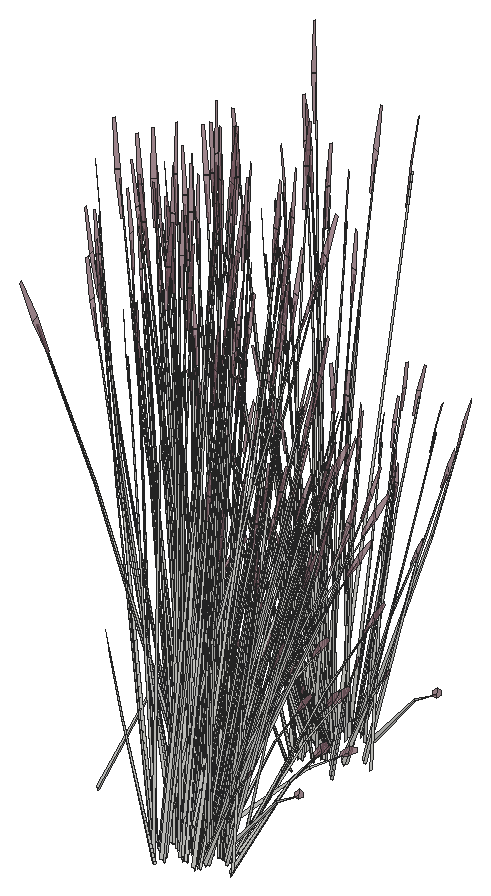
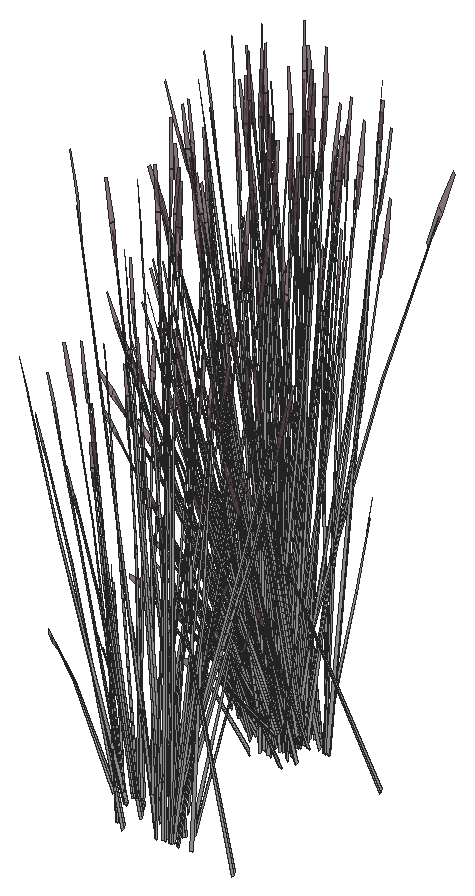
# SketchUp Ruby script. Lengths in inches.
U = 1.inch
M = Sketchup.active_model
def pt(a) = Geom::Point3d.new(a.map { |v| v * U })
def face(e, loops, mat)
  f = e.add_face(loops[0].map { |a| pt(a) })
  loops[1..].each { |l| e.add_face(l.map { |a| pt(a) }).erase! }
  f.material = f.back_material = mat if mat
  f
end
# faces: each face lists its corners as indices into pts; further lists are holes
def faces(e, pts, list, mat = nil) = list.each { |f| face(e, (f[0].is_a?(Array) ? f : [f]).map { |l| l.map { |i| pts[i] } }, mat) }
# xy, xz, yz: faces in a plane at the given z, y or x. An outline is a flat list of corners, or four numbers for a rectangle; further outlines are holes
def ring(l) = l.size == 4 ? [[l[0], l[1]], [l[2], l[1]], [l[2], l[3]], [l[0], l[3]]] : l.each_slice(2).to_a
def flat(e, list, mat, &to3) = list.each { |f| face(e, (f[0].is_a?(Array) ? f : [f]).map { |l| ring(l).map { |u, v| to3.(u, v) } }, mat) }
def xy(e, z, list, mat = nil) = flat(e, list, mat) { |x, y| [x, y, z] }
def xz(e, y, list, mat = nil) = flat(e, list, mat) { |x, z| [x, y, z] }
def yz(e, x, list, mat = nil) = flat(e, list, mat) { |y, z| [x, y, z] }
def lines(e, pts, list) = list.each { |a, b| e.add_line(pt(pts[a]), pt(pts[b])) }
# prism: a flat outline (further loops are holes) pulled along v
def prism(e, loops, v, mat = nil)
  f = face(e, loops, mat); d = Geom::Vector3d.new(v.map { |x| x * U })
  f.pushpull(f.normal.samedirection?(d) ? d.length : -d.length)
end
def box(e, o, s, mat = nil) = prism(e, [[o, [o[0] + s[0], o[1], o[2]], [o[0] + s[0], o[1] + s[1], o[2]], [o[0], o[1] + s[1], o[2]]]], [0, 0, s[2]], mat)
def at(x, y, z, deg = 0) = Geom::Transformation.translation(pt([x, y, z])) * Geom::Transformation.rotation(ORIGIN, Z_AXIS, deg.degrees)
def axes(o, x, y, z) = Geom::Transformation.new([*x, 0, *y, 0, *z, 0, *pt(o).to_a, 1])
def part(name) = M.definitions.add(name)
# library, detail: a bought-in or finely detailed component or shape, given as its bounding box
def library(name, o, s) = part(name).tap { |d| box(d.entities, o, s) }
def detail(e, o, s) = box(e.add_group.entities, o, s)
def put(e, d, t, mat = nil) = e.add_instance(d, t).tap { |i| i.material = mat if mat }
def group(e, t, mat = nil) = e.add_group.tap { |g| g.transformation = t; g.material = mat if mat }.entities
root = M.entities
M.materials.add("LightPink_Translucent").color = [144, 107, 117]
M.materials["LightPink_Translucent"].alpha = 0.75
c1 = part("blade")
p = [[2.15,0.21,22],[0,0.17,0],[0.09,0.45,0],[2.18,0.31,22],[2.29,0.31,22],[0.38,0.45,0],
  [2.48,0.24,33],[2.49,0.24,33],[2.48,0.22,33]]
faces(c1.entities,p,[[0,1,2,3],[4,5,2,3],[6,3,4,7],[8,0,3,6]])
c2 = part("seeds")
p = [[0.3,-0.1,1.38],[-0.01,-0.03,1.59],[-0.01,-0.03,0.03],[0.14,-0.07,-0.07],[0.29,-0.03,3],[0.15,0.01,3.11]]
faces(c2.entities,p,[[0,1,2,3],[1,0,4,5]],"LightPink_Translucent")
c3 = part("blade with seeds")
put(c3.entities,c1,at(0,0,0))
put(c3.entities,c2,axes([2.4,0.25,30.99],[1.5799,-0.05474,1.17369],[-0.12525,1.92788,0.29478],[-0.07173,-0.02425,1.56792]))
put(root,c3,axes([506.375,142.96,1.57],[-0.47504,-0.61229,0],[0.79476,-0.34146,-0.51607],[0.18101,-0.07777,1.63711]))
put(root,c3,axes([510.65,144.14,3.875],[-0.19519,-0.55794,-0.51099],[0.73919,-0.0976,-0.3958],[0.21183,-0.14986,0.97773]))
put(root,c3,axes([507.42,142.22,1.32],[-0.52505,0.35054,-0.03893],[-0.48109,-0.38392,-0.17649],[-0.03387,-0.10878,0.58215]))
put(root,c3,axes([510.99,144.54,4.23],[-0.70283,-0.33692,-0.1216],[0.40491,-0.48793,-0.67495],[0.19857,-0.16961,1.02557]))
put(root,c3,axes([508.09,146.38,2.52],[0.65659,0.2464,1.51261],[-0.64324,0.53082,0.59816],[-0.28812,-0.31461,1.26806]))
put(root,c3,axes([504.66,144.68,1.21],[0,-0.61104,-0.49651],[0.85008,0,0],[0,-0.13917,1.57504]))
put(root,c3,axes([507.02,142.87,1.21],[0.7111,-0.30552,-0.49651],[0.42504,0.54784,0],[0.16196,-0.06958,1.57504]))
put(root,c3,axes([511.24,143.92,1.78],[-0.27143,-0.0181,1.43002],[-0.27808,-0.48551,-0.30754],[0.33346,-0.13735,0.61141]))
put(root,c3,axes([512.72,144.39,3.9],[-0.09924,-0.00464,1.77383],[-0.4121,-0.49725,-0.16761],[0.1655,-0.1635,0.31391]))
put(root,c3,axes([507.86,144.12,1.25],[0.51177,-0.45928,-0.62353],[0.63575,0.41646,-0.16365],[0.20507,-0.11457,1.37633]))
put(root,c3,axes([511.55,143.03,1.96],[-0.25308,0.31105,1.1486],[-0.21753,-0.4179,0.84392],[0.20902,-0.10472,0.25299]))
put(root,c3,axes([511.19,144.2,3.72],[0.66138,-0.08733,-0.35414],[0.17464,0.49921,0.4572],[0.18953,-0.13408,0.87481]))
put(root,c3,axes([506.97,144.93,1.4],[0.36864,-0.55059,-0.44739],[0.76598,0.26498,0.21531],[0,-0.12692,1.43643]))
put(root,c3,axes([507.31,144.65,1.86],[-0.08854,-0.69723,-0.29095],[0.92215,-0.04216,-0.50002],[0.16238,-0.09287,1.59708]))
put(root,c3,axes([505.02,144.69,1.22],[0.53038,-0.38124,-0.30978],[0.53038,0.38124,0.30978],[0,-0.1228,1.38974]))
put(root,c3,axes([510.65,144.49,4.24],[-0.66138,0.08733,0.35414],[-0.17464,-0.49921,-0.4572],[0.18953,-0.13408,0.87481]))
put(root,c3,axes([506.88,145.38,1.86],[-0.85568,-0.29155,-0.29095],[0.41201,-0.61537,-0.50002],[-0.02689,-0.15109,1.59708]))
put(root,c3,axes([507.1875,143.11,1.22],[0.70886,0.15119,-0.30978],[-0.17848,0.53243,0.30978],[0.1429,-0.0614,1.38974]))
put(root,c3,axes([511.25,144.42,3.92],[0.52161,0.25698,0.0643],[-0.30368,0.36595,0.50621],[0.16723,-0.11831,0.77189]))
put(root,c3,axes([511.11,144.31,3.93],[0.18844,0.56237,0.48003],[-0.73919,0.0976,0.3958],[0.21785,-0.13226,0.9933]))
put(root,c3,axes([513.1,144.99,3.91],[0.10543,-0.09307,1.74944],[-0.13495,-0.57092,-0.27667],[0.26455,-0.10825,0.14031]))
put(root,c3,axes([505.18,144.96,1.52],[-0.70674,0.51372,0.30756],[-0.70717,-0.50832,-0.36492],[-0.02468,-0.14589,1.64885]))
put(root,c3,axes([507.43,145.2,1.625],[0.8561,0.29616,0.24065],[-0.41201,0.61537,0.50002],[0,-0.14185,1.60543]))
put(root,c3,axes([507.1,146.03,1.63],[0.20138,-0.72405,-0.23429],[0.95485,0.12621,0.51271],[-0.16685,-0.09999,1.5644]))
put(root,c3,axes([507.15,144.79,1.91],[-0.82508,0.03772,0.44739],[-0.07462,-0.62614,-0.21531],[0.14771,-0.06346,1.43643]))
put(root,c3,axes([505.02,145.24,1.67],[0,0.61104,0.49651],[-0.85008,0,0],[0,-0.13917,1.57504]))
put(root,c3,axes([511.02,145.86,4.23],[-0.38229,-0.5533,-0.1216],[0.6785,-0.2719,-0.67495],[0.28593,-0.073,1.02557]))
put(root,c3,axes([510.99,145.38,3.875],[0.20584,-0.55581,-0.51099],[0.70573,0.19051,-0.3958],[0.28414,-0.05097,0.97773]))
put(root,c3,axes([509.875,143.12,1.57],[0.47504,-0.61229,0],[0.79476,0.34146,-0.51607],[0.18101,0.07777,1.63711]))
put(root,c3,axes([507.03,145.74,1.4],[-0.45644,-0.51287,-0.44739],[0.69137,-0.36116,0.21531],[-0.14771,-0.06346,1.43643]))
put(root,c3,axes([507.125,145.01,1.55],[0.33034,0.68327,0.45755],[-0.94388,0.2376,0.17955],[0.01154,-0.12555,1.58856]))
put(root,c3,axes([511.74,145.54,1.17],[-0.48937,0.07333,1.41583],[-0.07789,-0.58369,0.08104],[0.34275,-0.08835,0.80566]))
put(root,c3,axes([512.63,145.02,1.45],[-0.47106,-0.39072,-0.06488],[0.51591,-0.35801,-0.29416],[0.14618,-0.02521,0.97024]))
put(root,c3,axes([506.96,145.55,1.91],[-0.36864,0.55059,0.44739],[-0.76598,-0.26498,-0.21531],[0,-0.12692,1.43643]))
put(root,c3,axes([508.3125,145.07,1.4],[0,-0.70701,0],[0.95008,0,0],[0,0,1.79456]))
put(root,c3,axes([509.46,143.4375,1.67],[-0.7111,-0.30552,0.49651],[0.42504,-0.54784,0],[0.16196,0.06958,1.57504]))
put(root,c3,axes([510.85,145.58,4.17],[0.66765,-0.26986,-0.71045],[0.37208,0.55551,0.08574],[0.32259,-0.0631,1.00501]))
put(root,c3,axes([507.86,144.625,1.55],[-0.62999,0.55453,0.45755],[-0.74845,-0.4895,0.17955],[0.15188,-0.05534,1.58856]))
put(root,c3,axes([508.55,145.62,1.49],[-0.70674,-0.52593,-0.06131],[0.70717,-0.52625,0],[-0.02468,-0.01837,1.75571]))
put(root,c3,axes([506.77,143.71,1.67],[-0.21949,0.60727,0.17642],[-0.8032,-0.17185,0.35086],[0.13875,-0.00296,1.60407]))
put(root,c3,axes([510.76,145.6875,4.24],[-0.63144,-0.17046,0.35414],[0.18417,-0.49731,-0.4572],[0.25423,-0.0456,0.87481]))
put(root,c3,axes([506.4375,144.2,0.79],[-0.74787,0.24464,1.28929],[-0.23804,-0.70192,0.50096],[0.45924,0.01168,1.46642]))
put(root,c3,axes([508.45,144.39,1.81],[0.14658,-0.54532,0.1448],[0.71613,0.09466,-0.41347],[0.13033,0.05599,1.26744]))
put(root,c3,axes([507.21,145.68,1.55],[0.96033,0.12874,0.45755],[-0.19544,0.7271,0.17955],[-0.14034,-0.07021,1.58856]))
put(root,c3,axes([512.28,145.16,0.6875],[-0.03971,-0.09277,1.76342],[0.27541,-0.54264,-0.26939],[0.27782,-0.00781,0.30037]))
put(root,c3,axes([508.14,144.53,1.91],[-0.45644,-0.51287,0.44739],[0.69137,-0.36116,-0.21531],[0.14771,0.06346,1.43643]))
put(root,c3,axes([506.69,146.84,1.67],[0.81646,-0.16218,0.17642],[0.20161,0.60355,0.35086],[-0.07282,-0.08794,1.60407]))
put(root,c3,axes([508.37,144.5625,1.86],[0.76714,-0.40567,-0.29095],[0.51013,0.57321,-0.50002],[0.18927,0.05821,1.59708]))
put(root,c3,axes([511.42,145.63,3.72],[0.63144,0.17046,-0.35414],[-0.18417,0.49731,0.4572],[0.25423,-0.0456,0.87481]))
put(root,c3,axes([510.31,143.49,1.21],[0.7111,0.30552,-0.49651],[-0.42504,0.54784,0],[0.16196,0.06958,1.57504]))
put(root,c3,axes([508.96,145.23,1.4],[0.85008,0,0],[0,0.63259,0],[0,0,1.78407]))
put(root,c3,axes([509.2,143.74,1.67],[-0.81646,0.16218,0.17642],[-0.20161,-0.60355,0.35086],[0.07282,0.08794,1.60407]))
put(root,c3,axes([509.7,145.02,3.07],[-0.31515,0.01384,1.71376],[0.20907,-0.5998,0.13857],[0.44912,0.0371,0.73262]))
put(root,c3,axes([510.11,143.71,1.22],[0.17848,0.53243,-0.30978],[-0.70886,0.15119,0.30978],[0.1429,0.0614,1.38974]))
put(root,c3,axes([511.33,145.84,3.92],[0.27906,0.41663,0.0643],[-0.50888,0.20393,0.50621],[0.22432,-0.04024,0.77189]))
put(root,c3,axes([508.68,144.91,1.57],[-0.96033,-0.12874,0.49198],[0.19544,-0.7271,0.19306],[0.14034,0.07021,1.70813]))
put(root,c3,axes([511.28,145.7,3.93],[-0.21466,0.55714,0.48003],[-0.70573,-0.19051,0.3958],[0.27753,-0.03348,0.9933]))
put(root,c3,axes([507.92,146.7,1.4],[-0.24791,-0.5268,0],[0.70791,-0.18448,0],[0,0,1.54371]))
put(root,c3,axes([507.44,146.2,1.81],[-0.14658,0.54532,0.1448],[-0.71613,-0.09466,-0.41347],[-0.13033,-0.05599,1.26744]))
put(root,c3,axes([508.84,146.63,1.38],[0.79769,-0.20732,-0.19198],[0.2803,0.59721,0.00008],[0.08805,-0.02292,1.73897]))
put(root,c3,axes([509.12,146.875,1.67],[0.21949,-0.60727,0.17642],[0.8032,0.17185,0.35086],[-0.13875,0.00296,1.60407]))
put(root,c3,axes([508.9375,145.5,1.41],[0.53038,0.39469,0],[-0.53038,0.39469,0],[0,0,1.69266]))
put(root,c3,axes([510.375,145.33,1.67],[-0.59697,-0.44509,0.17642],[0.60159,-0.4317,0.35086],[-0.06593,0.0909,1.60407]))
put(root,c3,axes([509.27,144.66,1.25],[0.79037,0.10018,-0.62353],[-0.16679,0.61794,-0.16365],[0.23587,0.07488,1.37633]))
put(root,c3,axes([512.76,145.73,1.96],[-0.46945,0.10088,1.1486],[0.22097,-0.4169,0.84392],[0.24904,0.02853,0.25299]))
put(root,c3,axes([507.74,146.94,1.39],[-0.76598,-0.27433,0],[0.36864,-0.57001,0],[0,0,1.62707]))
put(root,c3,axes([508.38,146.21,1.66],[-0.74193,-0.49181,-0.25192],[0.6243,-0.55226,0.5513],[-0.19979,0.05753,1.68216]))
put(root,c3,axes([506.42,147.15,1.67],[0.7111,0.30552,0.49651],[-0.42504,0.54784,0],[-0.16196,-0.06958,1.57504]))
put(root,c3,axes([508.93,145.04,1.91],[0.36864,-0.55059,0.44739],[0.76598,0.26498,-0.21531],[0,0.12692,1.43643]))
put(root,c3,axes([512.54,147.5,3.9],[-0.0687,-0.05349,1.77383],[0.15029,-0.57341,-0.16761],[0.27062,-0.03664,0.31391]))
put(root,c3,axes([508.79,145.35,1.48],[0,0.70667,-0.05637],[-0.95008,0,0],[0,0.02221,1.79368]))
put(root,c3,axes([508.86,144.85,1.4],[0.45644,0.51287,-0.44739],[-0.69137,0.36116,0.21531],[0.14771,0.06346,1.43643]))
put(root,c3,axes([511.95,147.02,3.12],[-0.14542,-0.51365,-0.03492],[0.68734,-0.11809,-0.15832],[0.14353,0.03256,0.52218]))
put(root,c3,axes([510.16,147,4.23],[0.04068,-0.62141,-0.1216],[0.77029,0.01698,-0.67495],[0.29667,0.04317,1.02557]))
put(root,c3,axes([510.87,145.34,1.67],[0,-0.61104,0.49651],[0.85008,0,0],[0,0.13917,1.57504]))
put(root,c3,axes([508.74,145.8,1.91],[0.82508,-0.03772,0.44739],[0.07462,0.62614,-0.21531],[-0.14771,0.06346,1.43643]))
put(root,c3,axes([509.25,145.16,1.81],[0.70791,-0.1782,0.1448],[0.24791,0.50885,-0.41347],[0,0.11199,1.26744]))
put(root,c3,axes([510.05,146.76,4.24],[-0.43232,-0.38257,0.35414],[0.49364,-0.36215,-0.4572],[0.25081,0.0551,0.87481]))
put(root,c3,axes([508,146.11,1.4],[-0.82508,0.03772,-0.44739],[-0.07462,-0.62614,0.21531],[-0.14771,0.06346,1.43643]))
put(root,c3,axes([511.88,146.4,1.78],[-0.18299,-0.15028,1.43002],[0.23809,-0.49714,-0.30754],[0.37023,0.06735,0.61141]))
put(root,c3,axes([508.61,146.95,1.4],[0.76598,0.27433,0],[-0.36864,0.57001,0],[0,0,1.74954]))
put(root,c3,axes([510.83,146.63,3.91],[0.16299,-0.01033,1.74944],[0.44707,-0.47471,-0.27667],[0.28992,0.06266,0.14031]))
put(root,c3,axes([508.92,147.56,1.39],[-0.46912,-0.61443,-0.05142],[0.79476,-0.34146,0.51607],[-0.19584,0.0585,1.6363]))
put(root,c3,axes([508.75,146.07,1.81],[0.56134,0.36712,0.1448],[-0.46823,0.41419,-0.41347],[-0.13033,0.05599,1.26744]))
put(root,c3,axes([510.2,146.71,4.17],[0.75952,0.01471,-0.71045],[-0.05101,0.61953,0.08574],[0.32177,0.06538,1.00501]))
put(root,c3,axes([509.35,147.2,1.67],[0.7111,-0.30552,0.49651],[0.42504,0.54784,0],[-0.16196,0.06958,1.57504]))
put(root,c3,axes([508.34,146.72,1.48],[0.33034,0.70197,-0.06012],[-0.94388,0.24598,0],[0.01154,0.02451,1.72173]))
put(root,c3,axes([508.7,147.48,1.22],[-0.70886,-0.15119,-0.30978],[0.17848,-0.53243,0.30978],[-0.1429,0.0614,1.38974]))
put(root,c3,axes([511.44,145.45,1.57],[0.95008,0,0],[0,0.68292,-0.51607],[0,0.15554,1.63711]))
put(root,c3,axes([511.0625,145.8,1.39],[-0.94962,-0.00489,-0.04976],[0,-0.68292,0.49943],[-0.02984,0.15546,1.58352]))
put(root,c3,axes([509.01,145.21,1.86],[0.85568,0.29155,-0.29095],[-0.41201,0.61537,-0.50002],[0.02689,0.15109,1.59708]))
put(root,c3,axes([510.66,146.96,3.72],[0.43232,0.38257,-0.35414],[-0.49364,0.36215,0.4572],[0.25081,0.0551,0.87481]))
put(root,c3,axes([510.87,145.9,1.22],[-0.53038,0.38124,-0.30978],[-0.53038,-0.38124,0.30978],[0,0.1228,1.38974]))
put(root,c3,axes([508.58,145.94,1.86],[0.08854,0.69723,-0.29095],[-0.92215,0.04216,-0.50002],[-0.16238,0.09287,1.59708]))
put(root,c3,axes([510.4375,147.11,3.92],[-0.03826,0.46465,0.0643],[-0.57772,-0.01274,0.50621],[0.2213,0.04862,0.77189]))
put(root,c3,axes([508.92,145.66,1.4],[-0.36864,0.55059,-0.44739],[-0.76598,-0.26498,0.21531],[0,0.12692,1.43643]))
put(root,c3,axes([497.1875,147.83,1.78],[-0.18299,-0.15028,1.43002],[0.23809,-0.49714,-0.30754],[0.37023,0.06735,0.61141]))
put(root,c3,axes([510.49,146.96,3.93],[-0.56024,0.40262,0.48003],[-0.48318,-0.42758,0.3958],[0.26285,0.07427,0.9933]))
put(root,c3,axes([508.71,147.43,4.24],[-0.11735,-0.49217,0.35414],[0.67083,-0.12996,-0.4572],[0.18018,0.14104,0.87481]))
put(root,c3,axes([508.9375,147.24,1.52],[0.95122,0.19861,0.30756],[-0.23797,0.7099,-0.36492],[-0.15744,0.08885,1.64885]))
put(root,c3,axes([508.87,147.72,1.21],[-0.7111,0.30552,-0.49651],[-0.42504,-0.54784,0],[-0.16196,0.06958,1.57504]))
put(root,c3,axes([511.23,145.91,1.21],[0,0.61104,-0.49651],[-0.85008,0,0],[0,0.13917,1.57504]))
put(root,c3,axes([509.11,145.98,3.07],[-0.28223,-0.10528,1.71376],[0.58406,-0.44165,0.13857],[0.36402,0.19924,0.73262]))
put(root,c3,axes([509.16,144.59,3.67],[-0.65655,-0.31748,1.38283],[0.69326,-0.49431,0.59665],[0.21183,0.29789,1.33663]))
put(root,c3,axes([510.15,147.18,1.96],[-0.4278,-0.1757,1.1486],[0.5524,-0.17852,0.84392],[0.14899,0.15122,0.25299]))
put(root,c3,axes([508.65,147.68,4.23],[0.45276,-0.52302,-0.1216],[0.65568,0.30132,-0.67495],[0.22792,0.14777,1.02557]))
put(root,c3,axes([505.66,146.97,4.24],[0.5141,-0.32171,0.35414],[0.48666,0.36734,-0.4572],[-0.07405,0.18664,0.87481]))
put(root,c3,axes([509.51,147.625,1.57],[0.47504,0.61229,0],[-0.79476,0.34146,-0.51607],[-0.18101,0.07777,1.63711]))
put(root,c3,axes([508.06,148.11,3.9],[0.00225,-0.07398,1.77383],[0.65113,-0.32638,-0.16761],[0.22617,0.1165,0.31391]))
put(root,c3,axes([510.27,147.83,0.6875],[0.05536,-0.08822,1.76342],[0.69692,-0.25981,-0.26939],[0.21129,0.13447,0.30037]))
put(root,c3,axes([509.11,145.2,2.03],[-0.02076,-0.57531,1.41272],[0.93937,0.14913,0.59816],[-0.22217,0.31481,1.3335]))
put(root,c3,axes([509.35,145.83,1.29],[0.2786,0.55945,-0.69212],[-0.80253,0.20149,-0.18165],[0.03079,0.18945,1.52773]))
put(root,c3,axes([509.18,147.42,3.875],[0.74975,-0.14525,-0.51099],[0.13115,0.55007,-0.3958],[0.20138,0.15763,0.97773]))
put(root,c3,axes([507.1,147.5,4.24],[0.22906,-0.4699,0.35414],[0.66828,0.13705,-0.4572],[0.06128,0.18919,0.87481]))
put(root,c3,axes([510.22,147.98,1.86],[-0.48723,-0.01916,1.0506],[0.32177,-0.40701,0.58006],[0.19248,0.1446,0.8241]))
put(root,c3,axes([508.82,147.87,3.92],[-0.34533,0.38816,0.0643],[-0.49176,-0.22599,0.50621],[0.15898,0.12445,0.77189]))
put(root,c3,axes([508,149.18,4.84],[0.52505,-0.35054,-0.06488],[0.48109,0.38392,-0.29416],[0.03387,0.10878,0.97024]))
put(root,c3,axes([508.96,147.76,3.93],[-0.75571,0.14023,0.48003],[-0.13115,-0.55007,0.3958],[0.17773,0.16212,0.9933]))
put(root,c3,axes([508.63,146.99,1.78],[0.01341,-0.20255,1.43002],[0.64074,-0.22625,-0.30754],[0.1978,0.24243,0.61141]))
put(root,c3,axes([506.9,147.93,3.92],[-0.55987,0.20767,0.0643],[-0.27403,-0.37869,0.50621],[0.05407,0.16693,0.77189]))
put(root,c3,axes([505.34,147.0625,4.59],[0.83505,0.03027,-0.13498],[-0.02282,0.57322,-0.74919],[-0.05801,0.22077,1.13838]))
put(root,c3,axes([506.88,147.7,4.23],[0.74352,-0.28449,-0.1216],[0.36538,0.50492,-0.67495],[0.0981,0.21277,1.02557]))
put(root,c3,axes([507.1,147.89,4.26],[-0.74868,-0.15974,0.53283],[0.25601,-0.52518,0.43934],[0.04499,0.20653,1.10256]))
put(root,c3,axes([505.72,148.68,1.96],[-0.01966,-0.36332,1.1486],[0.49135,0.25914,0.84392],[-0.09663,0.17317,0.25299]))
put(root,c3,axes([507.02,147.8125,0.6875],[0.12297,-0.03325,1.76342],[0.73967,0.18301,-0.26939],[0.02163,0.20626,0.30037]))
put(root,c3,axes([505.91,147.28,4.2],[0.54391,0.41056,-0.5672],[-0.57458,0.35956,-0.43934],[-0.08276,0.2086,1.08528]))
put(root,c3,axes([505.32,147.9,2.02],[0.69024,-0.1082,0.06507],[0.15868,0.43593,-0.86304],[-0.04376,0.22067,0.7736]))
put(root,c3,axes([507.52,147.68,3.875],[0.7469,0.15318,-0.51099],[-0.25601,0.52518,-0.3958],[0.06849,0.21144,0.97773]))
put(root,c3,axes([507.94,146.59,3.07],[-0.17368,-0.19618,1.71376],[0.80256,-0.16516,0.13857],[0.18139,0.30799,0.73262]))
put(root,c3,axes([507.18,148,3.72],[-0.22906,0.4699,-0.35414],[-0.66828,-0.13705,0.4572],[0.06128,0.18919,0.87481]))
put(root,c3,axes([505.74,147.09,4.53],[-0.01977,0.56521,-0.7886],[-0.83252,-0.03796,0.09517],[-0.08786,0.23945,1.11556]))
put(root,c3,axes([503.5625,148.58,3.9],[0.0862,-0.03689,1.77383],[0.71245,0.24539,-0.16761],[-0.01674,0.20431,0.31391]))
put(root,c3,axes([506.52,146.69,3.07],[-0.0186,-0.23452,1.71376],[0.80601,0.15558,0.13857],[-0.04985,0.33422,0.73262]))
put(root,c3,axes([507.25,147.58,4.17],[0.36264,0.49684,-0.71045],[-0.74649,0.27689,0.08574],[0.0848,0.24006,1.00501]))
put(root,c3,axes([506.71,148.83,3.91],[0.09631,0.0984,1.74944],[0.77725,0.03866,-0.27667],[0.07816,0.217,0.14031]))
put(root,c3,axes([505.46,147.89,2.56],[0.01669,-0.31544,1.54345],[0.75083,0.16661,0.21329],[-0.06506,0.33618,0.72882]))
put(root,c3,axes([507.52,161.39,1.78],[-0.21597,0.12368,1.43002],[-0.64681,-0.21647,-0.30754],[0.1199,-0.26922,0.61141]))
put(root,c3,axes([506.54,161.82,4.17],[-0.36264,-0.49684,-0.71045],[0.74649,-0.27689,0.08574],[-0.0848,-0.24006,1.00501]))
put(root,c3,axes([505.91,160.72,0.6875],[-0.12744,0.02202,1.76342],[-0.70477,-0.24781,-0.26939],[0.01183,-0.2067,0.30037]))
put(root,c3,axes([508.05,162.3,4.17],[0.01977,-0.56521,-0.71045],[0.83252,0.03796,0.08574],[0.08786,-0.23945,1.00501]))
put(root,c3,axes([509.21,161.42,3.91],[-0.00733,-0.12161,1.74944],[-0.61946,-0.35147,-0.27667],[0.09577,-0.21306,0.14031]))
put(root,c3,axes([506.61,161.4,3.72],[0.22906,-0.4699,-0.35414],[0.66828,0.13705,0.4572],[-0.06128,-0.18919,0.87481]))
put(root,c3,axes([507.11,162.02,3.07],[-0.14147,0.21002,1.71376],[-0.59349,-0.43464,0.13857],[0.26773,-0.27089,0.73262]))
put(root,c3,axes([509.04,160.98,3.9],[-0.07716,0.04667,1.77383],[-0.75601,-0.15746,-0.16761],[-0.02737,-0.20368,0.31391]))
put(root,c3,axes([506.26,161.72,3.875],[-0.7469,-0.15318,-0.51099],[0.25601,-0.52518,-0.3958],[-0.06849,-0.21144,0.97773]))
put(root,c3,axes([506.73,160.4,1.96],[0.09747,0.35631,1.1486],[-0.54071,-0.19735,0.84392],[0.05818,-0.18244,0.25299]))
put(root,c3,axes([507.88,162.12,3.875],[-0.54391,-0.41056,-0.51099],[0.57458,-0.35956,-0.3958],[0.08276,-0.2086,0.97773]))
put(root,c3,axes([506.6875,161.5,3.93],[0.74868,0.15974,0.48003],[-0.25601,0.52518,0.3958],[-0.04499,-0.20653,0.9933]))
put(root,c3,axes([506.9,161.69,4.23],[-0.74352,0.28449,-0.1216],[-0.36538,-0.50492,-0.67495],[-0.0981,-0.21277,1.02557]))
put(root,c3,axes([508.45,162.33,4.23],[-0.83505,-0.03027,-0.1216],[0.02282,-0.57322,-0.67495],[0.05801,-0.22077,1.02557]))
put(root,c3,axes([508.39,161.96,3.72],[0.5141,-0.32171,-0.35414],[0.48666,0.36734,0.4572],[0.07405,-0.18664,0.87481]))
put(root,c3,axes([506.89,161.46,3.92],[0.55987,-0.20767,0.0643],[0.27403,0.37869,0.50621],[-0.05407,-0.16693,0.77189]))
put(root,c3,axes([504.86,163.68,1.29],[-0.31203,-0.62659,-0.69835],[0.89884,-0.22566,-0.18329],[-0.03449,-0.21218,1.54149]))
put(root,c3,axes([509.03,161.77,0.6875],[-0.11372,-0.04814,1.76342],[-0.29211,-0.53779,-0.26939],[0.19706,-0.14594,0.30037]))
put(root,c3,axes([506.68,161.89,4.24],[-0.22906,0.4699,0.35414],[-0.66828,-0.13705,-0.4572],[-0.06128,-0.18919,0.87481]))
put(root,c3,axes([508.39,162.09,3.93],[0.54105,0.41691,0.48003],[-0.57458,0.35956,0.3958],[0.0998,-0.1956,0.9933]))
put(root,c3,axes([508.59,162.13,3.92],[0.62439,0.02847,0.0643],[-0.01712,0.42991,0.50621],[0.06534,-0.16468,0.77189]))
put(root,c3,axes([508.12,162.42,4.24],[-0.5141,0.32171,0.35414],[-0.48666,-0.36734,-0.4572],[0.07405,-0.18664,0.87481]))
put(root,c3,axes([509.03,163.29,4.17],[0.39688,-0.48213,-0.71045],[0.69548,0.34264,0.08574],[0.23697,-0.17468,1.00501]))
put(root,c3,axes([504.74,161.88,1.57],[-0.47504,-0.61229,0],[0.79476,-0.34146,-0.51607],[0.18101,-0.07777,1.63711]))
put(root,c3,axes([509.01,163.0625,3.875],[-0.19519,-0.55794,-0.51099],[0.73919,-0.0976,-0.3958],[0.21183,-0.14986,0.97773]))
put(root,c3,axes([505.78,161.14,1.32],[-0.52505,0.35054,-0.03893],[-0.48109,-0.38392,-0.17649],[-0.03387,-0.10878,0.58215]))
put(root,c3,axes([509.36,163.46,4.23],[-0.70283,-0.33692,-0.1216],[0.40491,-0.48793,-0.67495],[0.19857,-0.16961,1.02557]))
put(root,c3,axes([505.38,161.79,1.21],[0.7111,-0.30552,-0.49651],[0.42504,0.54784,0],[0.16196,-0.06958,1.57504]))
put(root,c3,axes([509.6,162.84,1.78],[-0.27143,-0.0181,1.43002],[-0.27808,-0.48551,-0.30754],[0.33346,-0.13735,0.61141]))
put(root,c3,axes([511.09,163.3125,3.9],[-0.09924,-0.00464,1.77383],[-0.4121,-0.49725,-0.16761],[0.1655,-0.1635,0.31391]))
put(root,c3,axes([506.23,163.04,1.25],[0.51177,-0.45928,-0.62353],[0.63575,0.41646,-0.16365],[0.20507,-0.11457,1.37633]))
put(root,c3,axes([509.92,161.95,1.96],[-0.25308,0.31105,1.1486],[-0.21753,-0.4179,0.84392],[0.20902,-0.10472,0.25299]))
put(root,c3,axes([509.55,163.12,3.72],[0.66138,-0.08733,-0.35414],[0.17464,0.49921,0.4572],[0.18953,-0.13408,0.87481]))
put(root,c3,axes([505.33,163.85,1.4],[0.36864,-0.55059,-0.44739],[0.76598,0.26498,0.21531],[0,-0.12692,1.43643]))
put(root,c3,axes([505.67,163.57,1.86],[-0.08854,-0.69723,-0.29095],[0.92215,-0.04216,-0.50002],[0.16238,-0.09287,1.59708]))
put(root,c3,axes([503.38,163.61,1.22],[0.53038,-0.38124,-0.30978],[0.53038,0.38124,0.30978],[0,-0.1228,1.38974]))
put(root,c3,axes([509.01,163.41,4.24],[-0.66138,0.08733,0.35414],[-0.17464,-0.49921,-0.4572],[0.18953,-0.13408,0.87481]))
put(root,c3,axes([505.24,164.3,1.86],[-0.85568,-0.29155,-0.29095],[0.41201,-0.61537,-0.50002],[-0.02689,-0.15109,1.59708]))
put(root,c3,axes([505.55,162.03,1.22],[0.70886,0.15119,-0.30978],[-0.17848,0.53243,0.30978],[0.1429,-0.0614,1.38974]))
put(root,c3,axes([509.61,163.34,3.92],[0.52161,0.25698,0.0643],[-0.30368,0.36595,0.50621],[0.16723,-0.11831,0.77189]))
put(root,c3,axes([509.47,163.23,3.93],[0.18844,0.56237,0.48003],[-0.73919,0.0976,0.3958],[0.21785,-0.13226,0.9933]))
put(root,c3,axes([511.46,163.91,3.91],[0.10543,-0.09307,1.74944],[-0.13495,-0.57092,-0.27667],[0.26455,-0.10825,0.14031]))
put(root,c3,axes([505.79,164.12,1.625],[0.8561,0.29616,0.24065],[-0.41201,0.61537,0.50002],[0,-0.14185,1.60543]))
put(root,c3,axes([505.51,163.71,1.91],[-0.82508,0.03772,0.44739],[-0.07462,-0.62614,-0.21531],[0.14771,-0.06346,1.43643]))
put(root,c3,axes([509.39,164.78,4.23],[-0.38229,-0.5533,-0.1216],[0.6785,-0.2719,-0.67495],[0.28593,-0.073,1.02557]))
put(root,c3,axes([509.35,164.3,3.875],[0.20584,-0.55581,-0.51099],[0.70573,0.19051,-0.3958],[0.28414,-0.05097,0.97773]))
put(root,c3,axes([508.24,162.04,1.57],[0.47504,-0.61229,0],[0.79476,0.34146,-0.51607],[0.18101,0.07777,1.63711]))
put(root,c3,axes([505.49,163.93,1.55],[0.33034,0.68327,0.45755],[-0.94388,0.2376,0.17955],[0.01154,-0.12555,1.58856]))
put(root,c3,axes([510.11,164.46,1.17],[-0.48937,0.07333,1.41583],[-0.07789,-0.58369,0.08104],[0.34275,-0.08835,0.80566]))
put(root,c3,axes([511,163.9375,1.45],[-0.47106,-0.39072,-0.06488],[0.51591,-0.35801,-0.29416],[0.14618,-0.02521,0.97024]))
put(root,c3,axes([498.16,165.49,1.78],[-0.27143,-0.0181,1.43002],[-0.27808,-0.48551,-0.30754],[0.33346,-0.13735,0.61141]))
put(root,c3,axes([505.32,164.47,1.91],[-0.36864,0.55059,0.44739],[-0.76598,-0.26498,-0.21531],[0,-0.12692,1.43643]))
put(root,c3,axes([506.67,163.99,1.4],[0,-0.70701,0],[0.95008,0,0],[0,0,1.79456]))
put(root,c3,axes([507.83,162.36,1.67],[-0.7111,-0.30552,0.49651],[0.42504,-0.54784,0],[0.16196,0.06958,1.57504]))
put(root,c3,axes([509.22,164.5,4.17],[0.66765,-0.26986,-0.71045],[0.37208,0.55551,0.08574],[0.32259,-0.0631,1.00501]))
